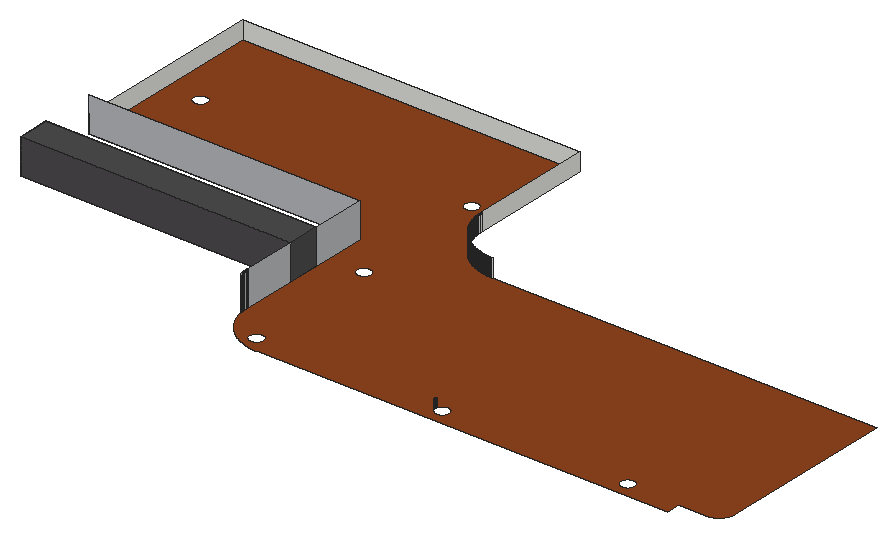
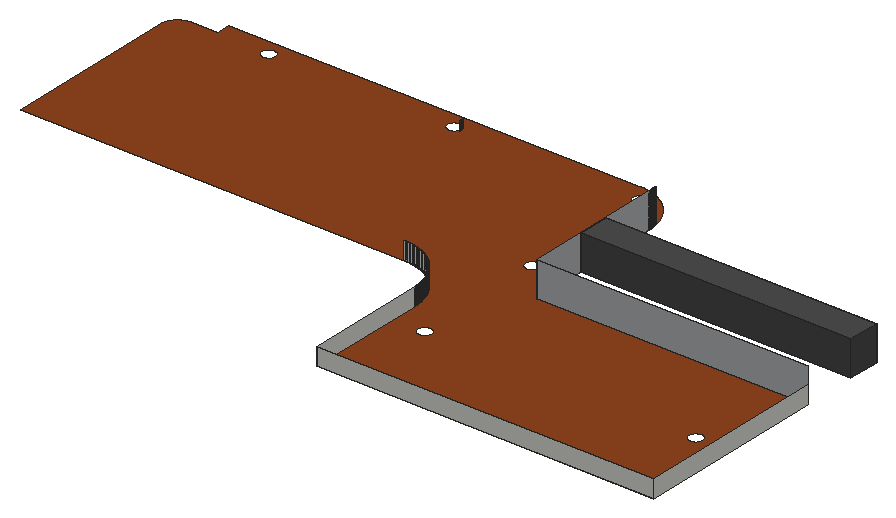
# SketchUp Ruby script. Lengths in inches.
U = 1.inch
M = Sketchup.active_model
def pt(a) = Geom::Point3d.new(a.map { |v| v * U })
def face(e, loops, mat)
  f = e.add_face(loops[0].map { |a| pt(a) })
  loops[1..].each { |l| e.add_face(l.map { |a| pt(a) }).erase! }
  f.material = f.back_material = mat if mat
  f
end
# faces: each face lists its corners as indices into pts; further lists are holes
def faces(e, pts, list, mat = nil) = list.each { |f| face(e, (f[0].is_a?(Array) ? f : [f]).map { |l| l.map { |i| pts[i] } }, mat) }
# xy, xz, yz: faces in a plane at the given z, y or x. An outline is a flat list of corners, or four numbers for a rectangle; further outlines are holes
def ring(l) = l.size == 4 ? [[l[0], l[1]], [l[2], l[1]], [l[2], l[3]], [l[0], l[3]]] : l.each_slice(2).to_a
def flat(e, list, mat, &to3) = list.each { |f| face(e, (f[0].is_a?(Array) ? f : [f]).map { |l| ring(l).map { |u, v| to3.(u, v) } }, mat) }
def xy(e, z, list, mat = nil) = flat(e, list, mat) { |x, y| [x, y, z] }
def xz(e, y, list, mat = nil) = flat(e, list, mat) { |x, z| [x, y, z] }
def yz(e, x, list, mat = nil) = flat(e, list, mat) { |y, z| [x, y, z] }
def lines(e, pts, list) = list.each { |a, b| e.add_line(pt(pts[a]), pt(pts[b])) }
# prism: a flat outline (further loops are holes) pulled along v
def prism(e, loops, v, mat = nil)
  f = face(e, loops, mat); d = Geom::Vector3d.new(v.map { |x| x * U })
  f.pushpull(f.normal.samedirection?(d) ? d.length : -d.length)
end
def box(e, o, s, mat = nil) = prism(e, [[o, [o[0] + s[0], o[1], o[2]], [o[0] + s[0], o[1] + s[1], o[2]], [o[0], o[1] + s[1], o[2]]]], [0, 0, s[2]], mat)
def at(x, y, z, deg = 0) = Geom::Transformation.translation(pt([x, y, z])) * Geom::Transformation.rotation(ORIGIN, Z_AXIS, deg.degrees)
def axes(o, x, y, z) = Geom::Transformation.new([*x, 0, *y, 0, *z, 0, *pt(o).to_a, 1])
def part(name) = M.definitions.add(name)
# library, detail: a bought-in or finely detailed component or shape, given as its bounding box
def library(name, o, s) = part(name).tap { |d| box(d.entities, o, s) }
def detail(e, o, s) = box(e.add_group.entities, o, s)
def put(e, d, t, mat = nil) = e.add_instance(d, t).tap { |i| i.material = mat if mat }
def group(e, t, mat = nil) = e.add_group.tap { |g| g.transformation = t; g.material = mat if mat }.entities
root = M.entities
M.materials.add("1423 AP 8230 BENTONITE").color = [77, 75, 77]
M.materials.add("1427 AP 686 ARMOUR-N").color = [184, 186, 189]
M.materials.add("[Wood Fence]").color = [142, 67, 30]
box(root,[18,156.5,366],[93,11,12],"1423 AP 8230 BENTONITE")
xy(root,366,[[[127.78,121,127.55,121.01,127.33,121.01,127.11,121.02,126.89,121.04,126.67,121.05,126.44,121.07,126.22,121.09,125.78,121.15,125.5625,121.18,125.34,121.21,125.12,121.25,124.9,121.28,124.68,121.33,124.47,121.37,124.03,121.47,123.82,121.52,123.6,121.58,123.39,121.64,123.17,121.7,122.96,121.76,122.54,121.9,122.33,121.98,122.12,122.05,121.49,122.29,121.09,122.47,120.88,122.5625,120.68,122.66,120.48,122.75,120.28,122.85,120.08,122.96,119.89,123.06,119.69,123.17,119.31,123.39,119.12,123.51,118.93,123.62,118.74,123.74,118.56,123.87,118.37,123.99,118.1875,124.12,118.01,124.25,117.65,124.51,117.48,124.65,117.3,124.79,116.96,125.07,116.79,125.22,116.46,125.52,116.14,125.82,115.82,126.14,115.52,126.46,115.22,126.79,115.07,126.96,114.79,127.3,114.65,127.48,114.51,127.65,114.25,128.01,114.12,128.1875,113.99,128.37,113.87,128.56,113.74,128.74,113.62,128.93,113.51,129.12,113.39,129.31,113.17,129.69,113.06,129.89,112.96,130.08,112.85,130.28,112.75,130.48,112.66,130.68,112.5625,130.88,112.47,131.09,112.29,131.49,112.05,132.12,111.98,132.33,111.9,132.54,111.76,132.96,111.7,133.17,111.64,133.39,111.58,133.6,111.52,133.82,111.47,134.03,111.37,134.47,111.33,134.68,111.28,134.9,111.25,135.12,111.21,135.34,111.18,135.5625,111.15,135.78,111.09,136.22,111.07,136.44,111.05,136.67,111.04,136.89,111.02,137.11,111.01,137.33,111.01,137.55,111,137.78,111,186,18,186,18,252,134,252,134,209.76,134.01,209.53,134.01,209.29,134.02,209.06,134.04,208.82,134.06,208.59,134.08,208.35,134.1,208.12,134.125,207.88,134.15,207.65,134.1875,207.42,134.22,207.18,134.3,206.72,134.35,206.49,134.39,206.26,134.44,206.03,134.5,205.8,134.55,205.57,134.61,205.34,134.68,205.11,134.74,204.89,134.81,204.66,134.88,204.4375,134.96,204.21,135.03,203.99,135.11,203.77,135.2,203.55,135.28,203.33,135.46,202.89,135.56,202.68,135.65,202.46,135.75,202.25,135.86,202.04,135.96,201.83,136.18,201.41,136.3,201.2,136.41,201,136.65,200.6,136.78,200.39,136.9,200.2,137.03,200,137.17,199.8,137.3,199.61,137.4375,199.42,137.58,199.23,137.72,199.04,137.86,198.86,138.01,198.67,138.16,198.49,138.3125,198.31,138.47,198.13,138.625,197.96,138.78,197.78,138.94,197.61,139.11,197.44,139.27,197.27,139.44,197.11,139.61,196.94,139.78,196.78,139.96,196.625,140.13,196.47,140.31,196.3125,140.49,196.16,140.67,196.01,140.86,195.86,141.04,195.72,141.23,195.58,141.42,195.4375,141.61,195.3,141.8,195.17,142,195.03,142.2,194.9,142.39,194.78,142.6,194.65,143,194.41,143.2,194.3,143.41,194.18,143.83,193.96,144.04,193.86,144.25,193.75,144.46,193.65,144.68,193.56,144.89,193.46,145.33,193.28,145.55,193.2,145.77,193.11,145.99,193.03,146.21,192.96,146.4375,192.88,146.66,192.81,146.89,192.74,147.11,192.68,147.34,192.61,147.57,192.55,147.8,192.5,148.03,192.44,148.26,192.39,148.49,192.35,148.72,192.3,149.18,192.22,149.42,192.1875,149.65,192.15,149.88,192.125,150.12,192.1,150.35,192.08,150.59,192.06,150.82,192.04,151.06,192.02,151.29,192.01,151.53,192.01,151.76,192,284,192,284,131.76,283.99,131.65,283.96,131.29,283.94,131.18,283.93,131.0625,283.91,130.95,283.88,130.83,283.86,130.71,283.83,130.6,283.81,130.49,283.77,130.37,283.71,130.15,283.67,130.03,283.63,129.92,283.59,129.8125,283.54,129.7,283.5,129.6,283.4,129.38,283.35,129.28,283.29,129.17,283.23,129.07,283.18,128.97,283.12,128.87,283.05,128.77,282.99,128.67,282.85,128.47,282.71,128.29,282.64,128.19,282.5625,128.1,282.48,128.01,282.41,127.93,282.33,127.84,282.24,127.76,282.16,127.67,282.07,127.59,281.99,127.51,281.9,127.4375,281.81,127.36,281.71,127.29,281.53,127.15,281.33,127.01,281.23,126.95,281.13,126.88,281.03,126.82,280.93,126.77,280.83,126.71,280.72,126.65,280.62,126.6,280.4,126.5,280.3,126.46,280.1875,126.41,280.08,126.37,279.97,126.33,279.85,126.29,279.63,126.23,279.51,126.19,279.4,126.17,279.29,126.14,279.17,126.12,279.05,126.09,278.9375,126.07,278.82,126.06,278.71,126.04,278.35,126.01,278.24,126,269,126,269,121],[29.84,216.5,30.16,216.5,30.24,216.51,30.3125,216.52,30.39,216.53,30.47,216.54,30.55,216.56,30.62,216.58,30.7,216.6,30.77,216.62,30.85,216.65,30.99,216.71,31.0625,216.74,31.13,216.77,31.41,216.93,31.47,216.98,31.53,217.02,31.59,217.07,31.71,217.18,31.77,217.23,31.82,217.29,31.93,217.41,31.98,217.47,32.02,217.53,32.07,217.59,32.23,217.87,32.26,217.9375,32.29,218.01,32.35,218.15,32.38,218.23,32.4,218.3,32.42,218.38,32.44,218.45,32.46,218.53,32.47,218.61,32.48,218.6875,32.49,218.76,32.5,218.84,32.5,219.16,32.49,219.24,32.48,219.3125,32.47,219.39,32.46,219.47,32.44,219.55,32.42,219.62,32.4,219.7,32.38,219.77,32.35,219.85,32.29,219.99,32.26,220.0625,32.23,220.13,32.07,220.41,32.02,220.47,31.98,220.53,31.93,220.59,31.82,220.71,31.77,220.77,31.71,220.82,31.59,220.93,31.53,220.98,31.47,221.02,31.41,221.07,31.13,221.23,31.0625,221.26,30.99,221.29,30.85,221.35,30.77,221.38,30.7,221.4,30.62,221.42,30.55,221.44,30.47,221.46,30.39,221.47,30.3125,221.48,30.24,221.49,30.16,221.5,29.84,221.5,29.76,221.49,29.6875,221.48,29.61,221.47,29.53,221.46,29.45,221.44,29.38,221.42,29.3,221.4,29.23,221.38,29.15,221.35,29.01,221.29,28.9375,221.26,28.87,221.23,28.59,221.07,28.53,221.02,28.47,220.98,28.41,220.93,28.29,220.82,28.23,220.77,28.18,220.71,28.07,220.59,28.02,220.53,27.98,220.47,27.93,220.41,27.77,220.13,27.74,220.0625,27.71,219.99,27.65,219.85,27.62,219.77,27.6,219.7,27.58,219.62,27.56,219.55,27.54,219.47,27.53,219.39,27.52,219.3125,27.51,219.24,27.5,219.16,27.5,218.84,27.51,218.76,27.52,218.6875,27.53,218.61,27.54,218.53,27.56,218.45,27.58,218.38,27.6,218.3,27.62,218.23,27.65,218.15,27.71,218.01,27.74,217.9375,27.77,217.87,27.93,217.59,27.98,217.53,28.02,217.47,28.07,217.41,28.18,217.29,28.23,217.23,28.29,217.18,28.41,217.07,28.47,217.02,28.53,216.98,28.59,216.93,28.87,216.77,28.9375,216.74,29.01,216.71,29.15,216.65,29.23,216.62,29.3,216.6,29.38,216.58,29.45,216.56,29.53,216.54,29.61,216.53,29.6875,216.52,29.76,216.51],[123.09,124,123.41,124,123.49,124.01,123.5625,124.02,123.64,124.03,123.72,124.04,123.8,124.06,123.87,124.08,123.95,124.1,124.02,124.12,124.1,124.15,124.24,124.21,124.3125,124.24,124.38,124.27,124.66,124.43,124.72,124.48,124.78,124.52,124.84,124.57,124.96,124.68,125.02,124.73,125.07,124.79,125.18,124.91,125.23,124.97,125.27,125.03,125.32,125.09,125.48,125.37,125.51,125.4375,125.54,125.51,125.6,125.65,125.63,125.73,125.65,125.8,125.67,125.88,125.69,125.95,125.71,126.03,125.72,126.11,125.73,126.1875,125.74,126.26,125.75,126.34,125.75,126.66,125.74,126.74,125.73,126.8125,125.72,126.89,125.71,126.97,125.69,127.05,125.67,127.12,125.65,127.2,125.63,127.27,125.6,127.35,125.54,127.49,125.51,127.5625,125.48,127.63,125.32,127.91,125.27,127.97,125.23,128.03,125.18,128.09,125.07,128.21,125.02,128.27,124.96,128.32,124.84,128.43,124.78,128.48,124.72,128.52,124.66,128.57,124.38,128.73,124.3125,128.76,124.24,128.79,124.1,128.85,124.02,128.88,123.95,128.9,123.87,128.92,123.8,128.94,123.72,128.96,123.64,128.97,123.5625,128.98,123.49,128.99,123.41,129,123.09,129,123.01,128.99,122.9375,128.98,122.86,128.97,122.78,128.96,122.7,128.94,122.63,128.92,122.55,128.9,122.48,128.88,122.4,128.85,122.26,128.79,122.1875,128.76,122.12,128.73,121.84,128.57,121.78,128.52,121.72,128.48,121.66,128.43,121.54,128.32,121.48,128.27,121.43,128.21,121.32,128.09,121.27,128.03,121.23,127.97,121.18,127.91,121.02,127.63,120.99,127.5625,120.96,127.49,120.9,127.35,120.87,127.27,120.85,127.2,120.83,127.12,120.81,127.05,120.79,126.97,120.78,126.89,120.77,126.8125,120.76,126.74,120.75,126.66,120.75,126.34,120.76,126.26,120.77,126.1875,120.78,126.11,120.79,126.03,120.81,125.95,120.83,125.88,120.85,125.8,120.87,125.73,120.9,125.65,120.96,125.51,120.99,125.4375,121.02,125.37,121.18,125.09,121.23,125.03,121.27,124.97,121.32,124.91,121.43,124.79,121.48,124.73,121.54,124.68,121.66,124.57,121.72,124.52,121.78,124.48,121.84,124.43,122.12,124.27,122.1875,124.24,122.26,124.21,122.4,124.15,122.48,124.12,122.55,124.1,122.63,124.08,122.7,124.06,122.78,124.04,122.86,124.03,122.9375,124.02,123.01,124.01],[186.97,124,187.28,124,187.36,124.01,187.4375,124.02,187.52,124.03,187.59,124.04,187.75,124.08,187.82,124.1,187.9,124.12,187.97,124.15,188.05,124.18,188.12,124.21,188.1875,124.24,188.26,124.27,188.4,124.35,188.46,124.39,188.53,124.43,188.59,124.48,188.66,124.52,188.72,124.57,188.84,124.68,188.95,124.79,189.15,125.03,189.19,125.09,189.24,125.16,189.32,125.3,189.35,125.37,189.39,125.4375,189.42,125.51,189.48,125.65,189.5,125.73,189.53,125.8,189.55,125.88,189.56,125.95,189.58,126.03,189.59,126.11,189.61,126.1875,189.61,126.26,189.62,126.34,189.625,126.42,189.625,126.58,189.62,126.66,189.61,126.74,189.61,126.8125,189.59,126.89,189.58,126.97,189.56,127.05,189.55,127.12,189.53,127.2,189.5,127.27,189.48,127.35,189.42,127.49,189.39,127.5625,189.35,127.63,189.32,127.7,189.24,127.84,189.19,127.91,189.15,127.97,188.95,128.21,188.84,128.32,188.72,128.43,188.66,128.48,188.59,128.52,188.53,128.57,188.46,128.61,188.4,128.65,188.26,128.73,188.1875,128.76,188.12,128.79,188.05,128.82,187.97,128.85,187.9,128.88,187.82,128.9,187.75,128.92,187.59,128.96,187.52,128.97,187.4375,128.98,187.36,128.99,187.28,129,186.97,129,186.89,128.99,186.8125,128.98,186.73,128.97,186.66,128.96,186.5,128.92,186.43,128.9,186.35,128.88,186.28,128.85,186.2,128.82,186.13,128.79,186.0625,128.76,185.99,128.73,185.85,128.65,185.79,128.61,185.72,128.57,185.66,128.52,185.59,128.48,185.53,128.43,185.41,128.32,185.3,128.21,185.1,127.97,185.06,127.91,185.01,127.84,184.93,127.7,184.9,127.63,184.86,127.5625,184.83,127.49,184.77,127.35,184.75,127.27,184.72,127.2,184.7,127.12,184.69,127.05,184.67,126.97,184.66,126.89,184.64,126.8125,184.64,126.74,184.63,126.66,184.625,126.58,184.625,126.42,184.63,126.34,184.64,126.26,184.64,126.1875,184.66,126.11,184.67,126.03,184.69,125.95,184.7,125.88,184.72,125.8,184.75,125.73,184.77,125.65,184.83,125.51,184.86,125.4375,184.9,125.37,184.93,125.3,185.01,125.16,185.06,125.09,185.1,125.03,185.3,124.79,185.41,124.68,185.53,124.57,185.59,124.52,185.66,124.48,185.72,124.43,185.79,124.39,185.85,124.35,185.99,124.27,186.0625,124.24,186.13,124.21,186.2,124.18,186.28,124.15,186.35,124.12,186.43,124.1,186.5,124.08,186.66,124.04,186.73,124.03,186.8125,124.02,186.89,124.01],[250.84,124,251.16,124,251.24,124.01,251.3125,124.02,251.39,124.03,251.47,124.04,251.55,124.06,251.62,124.08,251.7,124.1,251.77,124.12,251.85,124.15,251.99,124.21,252.0625,124.24,252.13,124.27,252.41,124.43,252.47,124.48,252.53,124.52,252.59,124.57,252.71,124.68,252.77,124.73,252.82,124.79,252.93,124.91,252.98,124.97,253.02,125.03,253.07,125.09,253.23,125.37,253.26,125.4375,253.29,125.51,253.35,125.65,253.38,125.73,253.4,125.8,253.42,125.88,253.44,125.95,253.46,126.03,253.47,126.11,253.48,126.1875,253.49,126.26,253.49,126.34,253.5,126.42,253.5,126.58,253.49,126.66,253.49,126.74,253.48,126.8125,253.47,126.89,253.46,126.97,253.44,127.05,253.42,127.12,253.4,127.2,253.38,127.27,253.35,127.35,253.29,127.49,253.26,127.5625,253.23,127.63,253.07,127.91,253.02,127.97,252.98,128.03,252.93,128.09,252.82,128.21,252.77,128.27,252.71,128.32,252.59,128.43,252.53,128.48,252.47,128.52,252.41,128.57,252.13,128.73,252.0625,128.76,251.99,128.79,251.85,128.85,251.77,128.88,251.7,128.9,251.62,128.92,251.55,128.94,251.47,128.96,251.39,128.97,251.3125,128.98,251.24,128.99,251.16,129,250.84,129,250.76,128.99,250.6875,128.98,250.61,128.97,250.53,128.96,250.45,128.94,250.38,128.92,250.3,128.9,250.23,128.88,250.15,128.85,249.94,128.76,249.86,128.73,249.8,128.69,249.59,128.57,249.53,128.52,249.47,128.48,249.41,128.43,249.29,128.32,249.23,128.27,249.18,128.21,249.07,128.09,249.02,128.03,248.98,127.97,248.93,127.91,248.77,127.63,248.74,127.5625,248.71,127.49,248.65,127.35,248.62,127.27,248.6,127.2,248.58,127.12,248.56,127.05,248.54,126.97,248.53,126.89,248.52,126.8125,248.51,126.74,248.5,126.66,248.5,126.34,248.51,126.26,248.52,126.1875,248.53,126.11,248.54,126.03,248.56,125.95,248.58,125.88,248.6,125.8,248.62,125.73,248.65,125.65,248.71,125.51,248.74,125.4375,248.77,125.37,248.93,125.09,248.98,125.03,249.02,124.97,249.07,124.91,249.18,124.79,249.23,124.73,249.29,124.68,249.41,124.57,249.47,124.52,249.53,124.48,249.59,124.43,249.8,124.31,249.86,124.27,249.94,124.24,250.15,124.15,250.23,124.12,250.3,124.1,250.38,124.08,250.45,124.06,250.53,124.04,250.61,124.03,250.6875,124.02,250.76,124.01],[123.09,216.5,123.41,216.5,123.49,216.51,123.5625,216.52,123.64,216.53,123.72,216.54,123.8,216.56,123.87,216.58,123.95,216.6,124.02,216.62,124.1,216.65,124.24,216.71,124.3125,216.74,124.38,216.77,124.66,216.93,124.72,216.98,124.78,217.02,124.84,217.07,124.96,217.18,125.02,217.23,125.07,217.29,125.18,217.41,125.23,217.47,125.27,217.53,125.32,217.59,125.48,217.87,125.51,217.9375,125.54,218.01,125.6,218.15,125.63,218.23,125.65,218.3,125.67,218.38,125.69,218.45,125.71,218.53,125.72,218.61,125.73,218.6875,125.74,218.76,125.75,218.84,125.75,219.16,125.74,219.24,125.73,219.3125,125.72,219.39,125.71,219.47,125.69,219.55,125.67,219.62,125.65,219.7,125.63,219.77,125.6,219.85,125.54,219.99,125.51,220.0625,125.48,220.13,125.32,220.41,125.27,220.47,125.23,220.53,125.18,220.59,125.07,220.71,125.02,220.77,124.96,220.82,124.84,220.93,124.78,220.98,124.72,221.02,124.66,221.07,124.38,221.23,124.3125,221.26,124.24,221.29,124.1,221.35,124.02,221.38,123.95,221.4,123.87,221.42,123.8,221.44,123.72,221.46,123.64,221.47,123.5625,221.48,123.49,221.49,123.41,221.5,123.09,221.5,123.01,221.49,122.9375,221.48,122.86,221.47,122.78,221.46,122.7,221.44,122.63,221.42,122.55,221.4,122.48,221.38,122.4,221.35,122.26,221.29,122.1875,221.26,122.12,221.23,121.84,221.07,121.78,221.02,121.72,220.98,121.66,220.93,121.54,220.82,121.48,220.77,121.43,220.71,121.32,220.59,121.27,220.53,121.23,220.47,121.18,220.41,121.02,220.13,120.99,220.0625,120.96,219.99,120.9,219.85,120.87,219.77,120.85,219.7,120.83,219.62,120.81,219.55,120.79,219.47,120.78,219.39,120.77,219.3125,120.76,219.24,120.75,219.16,120.75,218.84,120.76,218.76,120.77,218.6875,120.78,218.61,120.79,218.53,120.81,218.45,120.83,218.38,120.85,218.3,120.87,218.23,120.9,218.15,120.96,218.01,120.99,217.9375,121.02,217.87,121.18,217.59,121.23,217.53,121.27,217.47,121.32,217.41,121.43,217.29,121.48,217.23,121.54,217.18,121.66,217.07,121.72,217.02,121.78,216.98,121.84,216.93,122.12,216.77,122.1875,216.74,122.26,216.71,122.4,216.65,122.48,216.62,122.55,216.6,122.63,216.58,122.7,216.56,122.78,216.54,122.86,216.53,122.9375,216.52,123.01,216.51],[123.09,170.25,123.41,170.25,123.49,170.26,123.5625,170.27,123.64,170.28,123.72,170.29,123.8,170.31,123.87,170.33,123.95,170.35,124.02,170.37,124.1,170.4,124.24,170.46,124.3125,170.49,124.38,170.52,124.66,170.68,124.72,170.73,124.78,170.77,124.84,170.82,124.96,170.93,125.02,170.98,125.07,171.04,125.18,171.16,125.23,171.22,125.27,171.28,125.32,171.34,125.48,171.62,125.51,171.6875,125.54,171.76,125.6,171.9,125.63,171.98,125.65,172.05,125.67,172.13,125.69,172.2,125.71,172.28,125.72,172.36,125.73,172.4375,125.74,172.51,125.75,172.59,125.75,172.91,125.74,172.99,125.73,173.0625,125.72,173.14,125.71,173.22,125.69,173.3,125.67,173.37,125.65,173.45,125.63,173.52,125.6,173.6,125.54,173.74,125.51,173.8125,125.48,173.88,125.32,174.16,125.27,174.22,125.23,174.28,125.18,174.34,125.07,174.46,125.02,174.52,124.96,174.57,124.84,174.68,124.78,174.73,124.72,174.77,124.66,174.82,124.38,174.98,124.3125,175.01,124.24,175.04,124.1,175.1,124.02,175.13,123.95,175.15,123.87,175.17,123.8,175.19,123.72,175.21,123.64,175.22,123.5625,175.23,123.49,175.24,123.41,175.25,123.09,175.25,123.01,175.24,122.9375,175.23,122.86,175.22,122.78,175.21,122.7,175.19,122.63,175.17,122.55,175.15,122.48,175.13,122.4,175.1,122.26,175.04,122.1875,175.01,122.12,174.98,121.84,174.82,121.78,174.77,121.72,174.73,121.66,174.68,121.54,174.57,121.48,174.52,121.43,174.46,121.32,174.34,121.27,174.28,121.23,174.22,121.18,174.16,121.02,173.88,120.99,173.8125,120.96,173.74,120.9,173.6,120.87,173.52,120.85,173.45,120.83,173.37,120.81,173.3,120.79,173.22,120.78,173.14,120.77,173.0625,120.76,172.99,120.75,172.91,120.75,172.59,120.76,172.51,120.77,172.4375,120.78,172.36,120.79,172.28,120.81,172.2,120.83,172.13,120.85,172.05,120.87,171.98,120.9,171.9,120.96,171.76,120.99,171.6875,121.02,171.62,121.18,171.34,121.23,171.28,121.27,171.22,121.32,171.16,121.43,171.04,121.48,170.98,121.54,170.93,121.66,170.82,121.72,170.77,121.78,170.73,121.84,170.68,122.12,170.52,122.1875,170.49,122.26,170.46,122.4,170.4,122.48,170.37,122.55,170.35,122.63,170.33,122.7,170.31,122.78,170.29,122.86,170.28,122.9375,170.27,123.01,170.26]]],"[Wood Fence]")
xz(root,186,[[18,366,111,378]],"1427 AP 686 ARMOUR-N")
xz(root,192,[[151.76,366,152,372]])
xz(root,192.01,[[151.29,366,151.53,372]])
xz(root,252,[[18,366,134,372]])
yz(root,18,[[186,366,252,372]])
yz(root,111,[[137.78,366,138,378],[138,366,186,378]],"1427 AP 686 ARMOUR-N")
yz(root,111.01,[[137.33,366,137.55,378]],"1427 AP 686 ARMOUR-N")
yz(root,134,[[209.76,366,210,372],[210,366,252,372]])
yz(root,134.01,[[209.29,366,209.53,372]])
yz(root,184.625,[[126.42,366,126.5,369],[126.5,366,126.58,369]])
yz(root,184.64,[[126.1875,366,126.26,369],[126.74,366,126.8125,369]])
p = [[184.7,125.88,366],[184.69,125.95,366],[184.69,125.95,369],[184.7,125.88,369],[184.67,126.03,366],[184.66,126.11,366],
  [184.66,126.11,369],[184.67,126.03,369],[184.64,126.1875,366],[184.64,126.1875,369],[184.63,126.34,366],[184.625,126.42,366],
  [184.625,126.42,369],[184.63,126.34,369],[184.64,126.26,366],[184.64,126.26,369],[184.625,126.58,366],[184.63,126.66,366],
  [184.63,126.66,369],[184.625,126.58,369],[184.64,126.74,366],[184.64,126.74,369],[184.64,126.8125,366],[184.66,126.89,366],
  [184.66,126.89,369],[184.64,126.8125,369],[184.67,126.97,366],[184.67,126.97,369],[184.69,127.05,366],[184.69,127.05,369],
  [111.25,135.12,366],[111.28,134.9,366],[111.28,134.9,378],[111.25,135.12,378],[111.21,135.34,366],[111.21,135.34,378],
  [111.18,135.5625,366],[111.18,135.5625,378],[111.15,135.78,366],[111.15,135.78,378],[111.12,136,366],[111.12,136,378],
  [111.09,136.22,366],[111.09,136.22,378],[111.07,136.44,366],[111.07,136.44,378],[111.05,136.67,366],[111.05,136.67,378],
  [111.04,136.89,366],[111.04,136.89,378],[111.02,137.11,366],[111.02,137.11,378],[111.01,137.33,366],[111.01,137.33,378],
  [111,137.78,366],[111.01,137.55,366],[111.01,137.55,378],[111,137.78,378],[150.59,192.06,372],[150.82,192.04,372],
  [150.82,192.04,366],[150.59,192.06,366],[151.06,192.02,372],[151.06,192.02,366],[151.29,192.01,372],[151.29,192.01,366],
  [151.53,192.01,372],[151.76,192,372],[151.76,192,366],[151.53,192.01,366],[149.65,192.15,372],[149.88,192.125,372],
  [149.88,192.125,366],[149.65,192.15,366],[150.12,192.1,372],[150.12,192.1,366],[150.35,192.08,372],[150.35,192.08,366],
  [148.95,192.26,372],[149.18,192.22,372],[149.18,192.22,366],[148.95,192.26,366],[149.42,192.1875,372],[149.42,192.1875,366],
  [148.26,192.39,372],[148.49,192.35,372],[148.49,192.35,366],[148.26,192.39,366],[148.72,192.3,372],[148.72,192.3,366],
  [147.8,192.5,372],[148.03,192.44,372],[148.03,192.44,366],[147.8,192.5,366],[147.57,192.55,372],[147.57,192.55,366],
  [147.11,192.68,372],[147.34,192.61,372],[147.34,192.61,366],[147.11,192.68,366],[146.66,192.81,372],[146.89,192.74,372],
  [146.89,192.74,366],[146.66,192.81,366],[146.4375,192.88,372],[146.4375,192.88,366],[146.21,192.96,372],[146.21,192.96,366],
  [145.77,193.11,372],[145.99,193.03,372],[145.99,193.03,366],[145.77,193.11,366],[145.55,193.2,372],[145.55,193.2,366],
  [145.33,193.28,372],[145.33,193.28,366],[145.11,193.37,372],[145.11,193.37,366],[144.89,193.46,372],[144.89,193.46,366],
  [144.68,193.56,372],[144.68,193.56,366],[144.46,193.65,372],[144.46,193.65,366],[144.25,193.75,372],[144.25,193.75,366],
  [144.04,193.86,372],[144.04,193.86,366],[143.83,193.96,372],[143.83,193.96,366],[143.62,194.07,372],[143.62,194.07,366],
  [143.41,194.18,372],[143.41,194.18,366],[143.2,194.3,372],[143.2,194.3,366],[143,194.41,372],[143,194.41,366],
  [142.8,194.53,372],[142.8,194.53,366],[142.6,194.65,372],[142.6,194.65,366],[142.39,194.78,372],[142.39,194.78,366],
  [142.2,194.9,372],[142.2,194.9,366],[142,195.03,372],[142,195.03,366],[141.8,195.17,372],[141.8,195.17,366],
  [141.61,195.3,372],[141.61,195.3,366],[141.42,195.4375,372],[141.42,195.4375,366],[141.23,195.58,372],[141.23,195.58,366],
  [141.04,195.72,372],[141.04,195.72,366],[140.86,195.86,372],[140.86,195.86,366],[140.67,196.01,372],[140.67,196.01,366],
  [140.49,196.16,372],[140.49,196.16,366],[140.31,196.3125,372],[140.31,196.3125,366],[140.13,196.47,372],[140.13,196.47,366],
  [139.96,196.625,372],[139.96,196.625,366],[139.78,196.78,372],[139.78,196.78,366],[139.61,196.94,372],[139.61,196.94,366],
  [139.44,197.11,372],[139.44,197.11,366],[139.27,197.27,372],[139.27,197.27,366],[139.11,197.44,372],[139.11,197.44,366],
  [138.94,197.61,372],[138.94,197.61,366],[138.78,197.78,372],[138.78,197.78,366],[138.625,197.96,372],[138.625,197.96,366],
  [138.47,198.13,372],[138.47,198.13,366],[138.3125,198.31,372],[138.3125,198.31,366],[138.16,198.49,372],[138.16,198.49,366],
  [138.01,198.67,372],[138.01,198.67,366],[137.86,198.86,372],[137.86,198.86,366],[137.72,199.04,372],[137.72,199.04,366],
  [137.58,199.23,372],[137.58,199.23,366],[137.4375,199.42,372],[137.4375,199.42,366],[137.3,199.61,372],[137.3,199.61,366],
  [137.17,199.8,372],[137.17,199.8,366],[137.03,200,372],[137.03,200,366],[136.9,200.2,372],[136.9,200.2,366],
  [136.78,200.39,372],[136.78,200.39,366],[136.65,200.6,372],[136.65,200.6,366],[136.53,200.8,372],[136.53,200.8,366],
  [136.41,201,372],[136.41,201,366],[136.3,201.2,372],[136.3,201.2,366],[136.18,201.41,372],[136.18,201.41,366],
  [136.07,201.62,372],[136.07,201.62,366],[135.96,201.83,372],[135.96,201.83,366],[135.86,202.04,372],[135.86,202.04,366],
  [135.75,202.25,372],[135.75,202.25,366],[135.65,202.46,372],[135.65,202.46,366],[135.56,202.68,372],[135.56,202.68,366],
  [135.46,202.89,372],[135.46,202.89,366],[135.37,203.11,372],[135.37,203.11,366],[135.28,203.33,372],[135.28,203.33,366],
  [135.2,203.55,372],[135.2,203.55,366],[135.11,203.77,372],[135.11,203.77,366],[135.03,203.99,372],[135.03,203.99,366],
  [134.96,204.21,372],[134.96,204.21,366],[134.88,204.4375,372],[134.88,204.4375,366],[134.81,204.66,372],[134.81,204.66,366],
  [134.74,204.89,372],[134.74,204.89,366],[134.68,205.11,372],[134.68,205.11,366],[134.61,205.34,372],[134.61,205.34,366],
  [134.55,205.57,372],[134.55,205.57,366],[134.5,205.8,372],[134.5,205.8,366],[134.44,206.03,372],[134.44,206.03,366],
  [134.39,206.26,372],[134.39,206.26,366],[134.35,206.49,372],[134.35,206.49,366],[134.3,206.72,372],[134.3,206.72,366],
  [134.26,206.95,372],[134.26,206.95,366],[134.22,207.18,372],[134.22,207.18,366],[134.1875,207.42,372],[134.1875,207.42,366],
  [134.15,207.65,372],[134.15,207.65,366],[134.125,207.88,372],[134.125,207.88,366],[134.1,208.12,372],[134.1,208.12,366],
  [134.08,208.35,372],[134.08,208.35,366],[134.06,208.59,372],[134.06,208.59,366],[134.04,208.82,372],[134.04,208.82,366],
  [134.02,209.06,372],[134.02,209.06,366],[134.01,209.29,372],[134.01,209.29,366],[134,209.76,372],[134.01,209.53,372],
  [134.01,209.53,366],[134,209.76,366]]
faces(root,p,[[0,1,2,3],[4,5,6,7],[1,4,7,2],[5,8,9,6],[10,11,12,13],[14,10,13,15],[16,17,18,19],[17,20,21,18],
  [22,23,24,25],[23,26,27,24],[26,28,29,27],[58,59,60,61],[59,62,63,60],[62,64,65,63],[66,67,68,69],[70,71,72,73],
  [71,74,75,72],[74,76,77,75],[76,58,61,77],[78,79,80,81],[79,82,83,80],[82,70,73,83],[84,85,86,87],[85,88,89,86],
  [88,78,81,89],[90,91,92,93],[91,84,87,92],[94,90,93,95],[96,97,98,99],[97,94,95,98],[100,101,102,103],[101,96,99,102],
  [104,100,103,105],[106,104,105,107],[108,109,110,111],[109,106,107,110],[112,108,111,113],[114,112,113,115],[116,114,115,117],[118,116,117,119],
  [120,118,119,121],[122,120,121,123],[124,122,123,125],[126,124,125,127],[128,126,127,129],[130,128,129,131],[132,130,131,133],[134,132,133,135],
  [136,134,135,137],[138,136,137,139],[140,138,139,141],[142,140,141,143],[144,142,143,145],[146,144,145,147],[148,146,147,149],[150,148,149,151],
  [152,150,151,153],[154,152,153,155],[156,154,155,157],[158,156,157,159],[160,158,159,161],[162,160,161,163],[164,162,163,165],[166,164,165,167],
  [168,166,167,169],[170,168,169,171],[172,170,171,173],[174,172,173,175],[176,174,175,177],[178,176,177,179],[180,178,179,181],[182,180,181,183],
  [184,182,183,185],[186,184,185,187],[188,186,187,189],[190,188,189,191],[192,190,191,193],[194,192,193,195],[196,194,195,197],[198,196,197,199],
  [200,198,199,201],[202,200,201,203],[204,202,203,205],[206,204,205,207],[208,206,207,209],[210,208,209,211],[212,210,211,213],[214,212,213,215],
  [216,214,215,217],[218,216,217,219],[220,218,219,221],[222,220,221,223],[224,222,223,225],[226,224,225,227],[228,226,227,229],[230,228,229,231],
  [232,230,231,233],[234,232,233,235],[236,234,235,237],[238,236,237,239],[240,238,239,241],[242,240,241,243],[244,242,243,245],[246,244,245,247],
  [248,246,247,249],[250,248,249,251],[252,250,251,253],[254,252,253,255],[256,254,255,257],[258,256,257,259],[260,258,259,261],[262,260,261,263],
  [264,262,263,265],[266,264,265,267],[268,266,267,269],[270,268,269,271],[272,270,271,273],[274,272,273,275],[276,274,275,277],[278,276,277,279],
  [280,278,279,281],[282,280,281,283],[284,282,283,285],[286,284,285,287],[288,286,287,289],[290,288,289,291],[292,293,294,295]])
faces(root,p,[[30,31,32,33],[34,30,33,35],[36,34,35,37],[38,36,37,39],[40,38,39,41],[42,40,41,43],[44,42,43,45],[46,44,45,47],
  [48,46,47,49],[50,48,49,51],[52,50,51,53],[54,55,56,57]],"1427 AP 686 ARMOUR-N")
